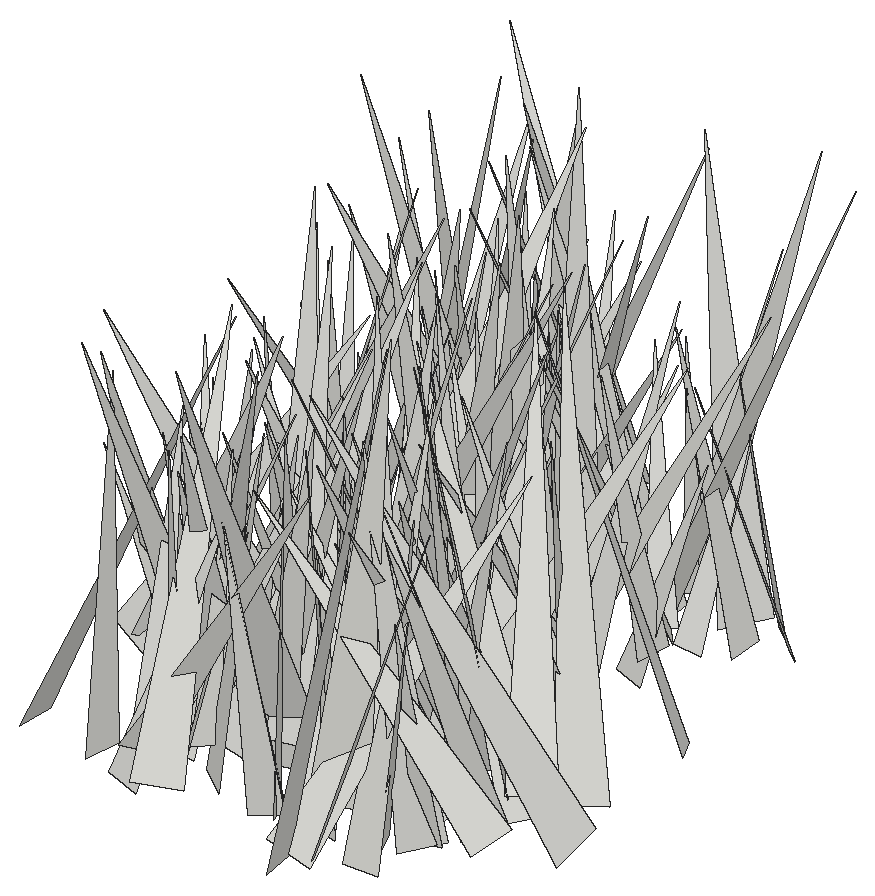
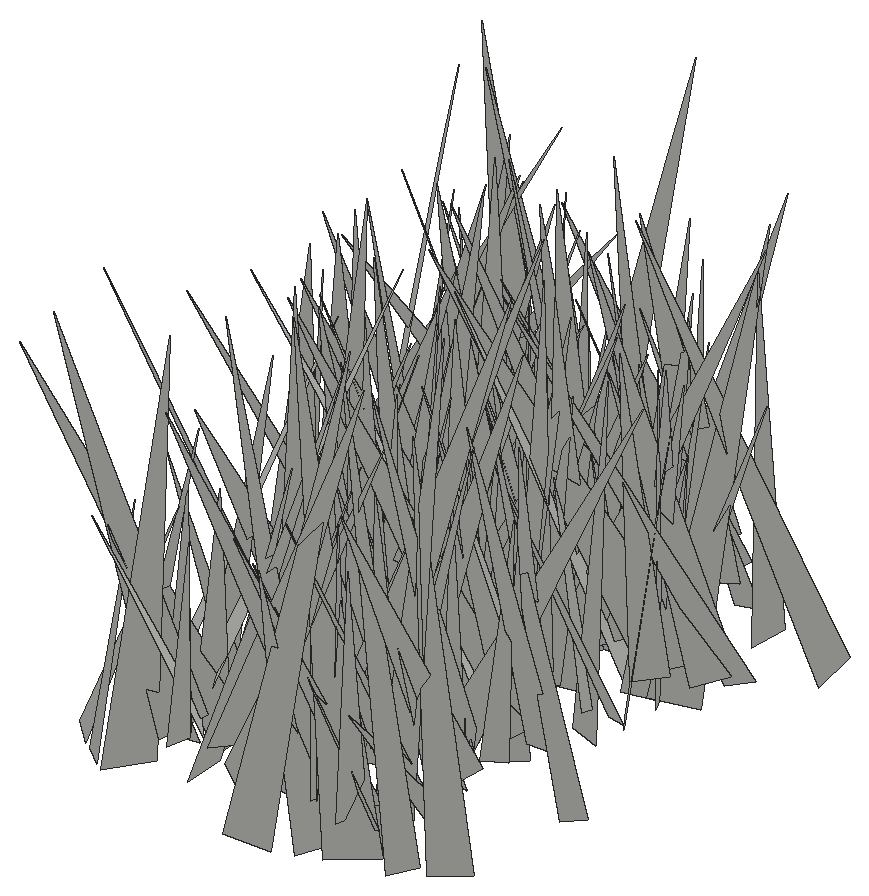
# SketchUp Ruby script. Lengths in inches.
U = 1.inch
M = Sketchup.active_model
def pt(a) = Geom::Point3d.new(a.map { |v| v * U })
def face(e, loops, mat)
  f = e.add_face(loops[0].map { |a| pt(a) })
  loops[1..].each { |l| e.add_face(l.map { |a| pt(a) }).erase! }
  f.material = f.back_material = mat if mat
  f
end
# faces: each face lists its corners as indices into pts; further lists are holes
def faces(e, pts, list, mat = nil) = list.each { |f| face(e, (f[0].is_a?(Array) ? f : [f]).map { |l| l.map { |i| pts[i] } }, mat) }
# xy, xz, yz: faces in a plane at the given z, y or x. An outline is a flat list of corners, or four numbers for a rectangle; further outlines are holes
def ring(l) = l.size == 4 ? [[l[0], l[1]], [l[2], l[1]], [l[2], l[3]], [l[0], l[3]]] : l.each_slice(2).to_a
def flat(e, list, mat, &to3) = list.each { |f| face(e, (f[0].is_a?(Array) ? f : [f]).map { |l| ring(l).map { |u, v| to3.(u, v) } }, mat) }
def xy(e, z, list, mat = nil) = flat(e, list, mat) { |x, y| [x, y, z] }
def xz(e, y, list, mat = nil) = flat(e, list, mat) { |x, z| [x, y, z] }
def yz(e, x, list, mat = nil) = flat(e, list, mat) { |y, z| [x, y, z] }
def lines(e, pts, list) = list.each { |a, b| e.add_line(pt(pts[a]), pt(pts[b])) }
# prism: a flat outline (further loops are holes) pulled along v
def prism(e, loops, v, mat = nil)
  f = face(e, loops, mat); d = Geom::Vector3d.new(v.map { |x| x * U })
  f.pushpull(f.normal.samedirection?(d) ? d.length : -d.length)
end
def box(e, o, s, mat = nil) = prism(e, [[o, [o[0] + s[0], o[1], o[2]], [o[0] + s[0], o[1] + s[1], o[2]], [o[0], o[1] + s[1], o[2]]]], [0, 0, s[2]], mat)
def at(x, y, z, deg = 0) = Geom::Transformation.translation(pt([x, y, z])) * Geom::Transformation.rotation(ORIGIN, Z_AXIS, deg.degrees)
def axes(o, x, y, z) = Geom::Transformation.new([*x, 0, *y, 0, *z, 0, *pt(o).to_a, 1])
def part(name) = M.definitions.add(name)
# library, detail: a bought-in or finely detailed component or shape, given as its bounding box
def library(name, o, s) = part(name).tap { |d| box(d.entities, o, s) }
def detail(e, o, s) = box(e.add_group.entities, o, s)
def put(e, d, t, mat = nil) = e.add_instance(d, t).tap { |i| i.material = mat if mat }
def group(e, t, mat = nil) = e.add_group.tap { |g| g.transformation = t; g.material = mat if mat }.entities
root = M.entities
c1 = part("fur_instance\#9")
p = [[0.8125,0,1.79],[0.67,-0.02,1.48],[0,-0.11,0],[0,0.11,0]]
faces(c1.entities,p,[[0,1,2,3]])
put(root,c1,axes([124.61,121.58,-28.22],[-3.04551,1.64304,1.0176],[0.80196,2.80235,-2.12461],[1.7584,1.56764,2.73144]))
put(root,c1,axes([126.19,110.12,-28.22],[-4.64353,0.24048,0.81476],[0.40253,4.60984,0.93348],[0.74809,-0.98772,4.55508]))
put(root,c1,axes([122.36,107.19,-28.22],[7.61599,0.93725,0.32253],[0.89381,-7.57423,0.90437],[-0.42844,0.85927,7.61996]))
put(root,c1,axes([124.81,111.45,-28.22],[2.89826,-6.60565,0.55734],[-6.55377,-2.94663,-0.84295],[-0.99662,0.16719,7.16407]))
put(root,c1,axes([122.79,118.57,-28.22],[-0.06945,-5.66946,1.63507],[-5.27402,0.7929,2.5253],[2.64594,1.43164,5.07647]))
put(root,c1,axes([125.08,106.82,-28.22],[5.69837,-0.41307,2.53776],[-0.52377,-6.22748,0.16244],[-2.51724,0.36068,5.71101]))
put(root,c1,axes([125.2,113.25,-28.22],[-3.34648,-2.86729,1.25208],[-2.75468,3.56945,0.81158],[1.4835,0.16004,4.33146]))
put(root,c1,axes([126.88,119.04,-27.1],[0.00181,-5.98408,0.19016],[-5.68264,-0.06159,-1.88392],[-1.88493,0.17992,5.67979]))
put(root,c1,axes([123.53,123.28,-28.22],[2.30675,-6.01681,0.97122],[-6.03702,-2.11321,1.24701],[0.83643,1.34116,6.32203]))
put(root,c1,axes([124.8,117.43,-27.1],[0.44242,5.64748,1.29703],[5.78226,-0.34572,-0.46699],[0.37666,-1.32609,5.6455]))
put(root,c1,axes([125.51,120.32,-27.1],[-5.11664,3.91829,0.85035],[3.38571,4.96082,-2.48663],[2.14782,1.51438,5.94556]))
put(root,c1,axes([125.24,111.59,-28.22],[-4.21315,-2.34987,2.26772],[-2.4638,4.71684,0.31027],[2.14339,0.80291,4.81418]))
put(root,c1,axes([125.67,120.82,-28.22],[4.21835,1.12148,1.8478],[0.48542,-4.44001,1.58659],[-2.10629,1.22277,4.06632]))
put(root,c1,axes([125.59,114.58,-28.22],[-1.84582,-5.09705,1.94608],[-5.40108,1.99766,0.10933],[0.77171,1.78987,5.41987]))
put(root,c1,axes([125.86,111.73,-28.22],[1.70929,-4.46495,1.67991],[-4.63149,-1.98085,-0.55231],[-1.1433,1.34907,4.74893]))
put(root,c1,axes([125.46,118.85,-27.1],[2.03457,-2.99845,1.01926],[-3.06758,-2.16697,-0.25148],[-0.78708,0.69471,3.61482]))
put(root,c1,axes([124.99,112.33,-27.1],[3.66382,-3.28739,1.57998],[-3.52995,-3.75957,0.36325],[-0.918,1.33625,4.90903]))
put(root,c1,axes([126.52,115.62,-28.22],[-0.46142,6.00885,1.03301],[6.04976,0.32253,0.82618],[-0.75742,-1.08443,5.96964]))
put(root,c1,axes([126.78,108.91,-28.22],[-3.90269,-1.36809,1.23152],[-1.73858,3.68797,-1.41263],[0.60468,1.77384,3.88679]))
put(root,c1,axes([126.83,109.45,-27.1],[-3.66348,3.88372,0.60062],[3.90017,3.69385,-0.09601],[0.48235,-0.37054,5.33808]))
put(root,c1,axes([126.3,116.91,-28.22],[-2.6188,2.85202,1.01974],[2.95253,2.70449,0.01846],[0.67563,-0.76402,3.87193]))
put(root,c1,axes([124.25,114.82,-27.1],[2.1149,3.97719,0.39309],[3.90996,-1.96694,-1.13523],[0.82754,-0.87089,4.35914]))
put(root,c1,axes([125.79,123.23,-28.22],[-1.04012,-7.65192,1.88155],[-7.84849,1.17518,0.4406],[0.70237,1.80029,7.70971]))
put(root,c1,axes([128.03,119.93,-27.1],[-6.43885,-0.2283,0.73687],[-0.34147,6.39798,-1.00159],[0.69173,1.03328,6.36457]))
put(root,c1,axes([123.48,125.51,-27.1],[7.4678,0.08394,0.57516],[0.2355,-7.21321,-2.00499],[-0.53141,-2.01703,7.1941]))
put(root,c1,axes([123.48,111.28,-27.1],[4.4628,-4.8312,0.78242],[-4.8199,-4.15484,1.83716],[0.84924,1.80724,6.31521]))
put(root,c1,axes([126.61,123.95,-27.1],[-4.17339,1.81444,1.20525],[1.74242,4.34394,-0.50613],[1.30721,0.0026,4.52253]))
put(root,c1,axes([122.82,110.91,-27.1],[1.506,6.6666,0.93752],[6.04421,-0.91584,-3.19677],[2.9648,-1.51928,6.04088]))
put(root,c1,axes([124.81,111.29,-27.1],[3.82808,-2.96393,0.87418],[-3.08142,-3.76593,0.72521],[-0.23226,1.11183,4.78677]))
put(root,c1,axes([126.13,119.27,-27.1],[6.62272,2.03005,2.53711],[1.31072,-6.93962,2.13125],[-2.97322,1.46257,6.59085]))
put(root,c1,axes([127.06,109.6,-27.1],[1.34944,-6.66989,1.0863],[-6.57389,-1.5523,-1.36482],[-1.56569,0.76902,6.66676]))
put(root,c1,axes([128.25,112.76,-28.22],[-6.66712,2.68909,2.42043],[3.53397,5.92752,3.14894],[0.77508,-3.89533,6.46266]))
put(root,c1,axes([126.89,109.55,-28.22],[4.42222,0.57042,2.59632],[0.96066,-5.04183,-0.52855],[-2.47858,-0.93641,4.42741]))
put(root,c1,axes([126.93,106.68,-27.1],[-2.07994,4.49979,1.08625],[4.57933,2.1742,-0.23818],[0.67657,-0.88257,4.95151]))
put(root,c1,axes([126.49,119.4,-27.1],[0.16475,-3.83195,1.51207],[-4.1166,-0.0965,0.20397],[0.15418,1.51796,3.83006]))
put(root,c1,axes([124.79,121.87,-28.22],[2.64419,5.03318,0.33977],[4.95036,-2.51506,-1.26831],[0.97076,-0.88412,5.54221]))
put(root,c1,axes([125.23,114.86,-27.1],[4.19489,0.81761,0.41517],[0.91291,-3.90671,-1.53042],[-0.08632,-1.58339,3.99042]))
put(root,c1,axes([129.45,120.01,-27.1],[-0.93338,-7.69941,2.7531],[-7.87622,0.10215,-2.38461],[-2.19672,2.90522,7.38009]))
put(root,c1,axes([125.91,117.17,-27.1],[4.66394,-1.20705,1.00362],[-1.36601,-4.67089,0.73033],[-0.77347,0.97077,4.76192]))
put(root,c1,axes([126.33,119.3,-27.1],[2.59266,-2.6088,0.97622],[-2.78019,-2.50569,0.68761],[-0.17141,1.18171,3.61316]))
put(root,c1,axes([126.4,123.89,-28.22],[2.97768,-2.23657,0.59018],[-2.29034,-2.98547,0.24174],[-0.32391,0.5494,3.71623]))
put(root,c1,axes([126.83,108.05,-28.22],[-0.69382,4.82103,0.91338],[4.82167,0.84094,-0.77604],[0.90996,-0.78004,4.80848]))
put(root,c1,axes([125.34,108.33,-28.22],[4.56915,3.9518,0.34933],[3.96081,-4.51383,-0.74378],[0.22516,-0.79028,5.99505]))
put(root,c1,axes([126.96,109.85,-27.1],[3.0521,-3.8403,0.46149],[-3.78154,-3.08617,-0.67208],[-0.8129,-0.06212,4.85917]))
put(root,c1,axes([128.1,120.41,-27.1],[-0.91047,5.0165,1.03079],[5.11456,0.83694,0.44447],[-0.2628,-1.09133,5.07905]))
put(root,c1,axes([127.37,114.76,-27.1],[5.69628,-2.00129,2.37758],[-1.98509,-6.1627,-0.4314],[-2.39112,0.34864,6.02217]))
put(root,c1,axes([127.39,123.42,-27.1],[4.14484,0.5886,1.74948],[0.68446,-4.48393,-0.11303],[-1.71425,-0.36717,4.1849]))
put(root,c1,axes([129.4,118.64,-28.22],[-1.28539,6.13898,3.44989],[6.89976,0.39684,1.86462],[-1.40785,-3.66012,5.98853]))
put(root,c1,axes([127.125,110.68,-28.22],[6.25178,5.32919,0.93445],[4.93149,-6.20008,2.36594],[-2.22574,1.23164,7.86685]))
put(root,c1,axes([128.85,110.96,-28.22],[-5.31707,5.30249,0.96243],[5.27581,5.39738,-0.58989],[1.09932,-0.2564,7.48596]))
put(root,c1,axes([128.19,115.38,-28.22],[1.47343,-6.07806,1.78682],[-6.21699,-1.74005,-0.79238],[-1.21846,1.52838,6.20371]))
put(root,c1,axes([128.37,113.5,-28.22],[0.55696,-4.64877,2.01019],[-4.98122,-0.86859,-0.62855],[-0.91614,1.89648,4.63963]))
put(root,c1,axes([126.89,121.04,-28.22],[4.28943,0.41298,0.87796],[0.18379,-4.25331,1.1028],[-0.95267,1.03894,4.16576]))
put(root,c1,axes([127.2,114.43,-27.1],[4.74802,-2.11154,0.82126],[-1.70244,-4.58339,-1.94189],[-1.49491,-1.48682,4.81989]))
put(root,c1,axes([127.65,107.01,-27.1],[-2.05605,-4.2865,1.82271],[-4.5186,2.31917,0.35698],[1.13077,1.47345,4.74068]))
put(root,c1,axes([128.4,107.31,-27.1],[-3.95695,1.67084,0.9926],[1.45221,4.03835,-1.00857],[1.29152,0.5783,4.17516]))
put(root,c1,axes([125.59,124.08,-27.1],[2.92691,3.10527,0.26779],[2.82947,-2.4932,-2.01476],[1.3071,-1.55642,3.76168]))
put(root,c1,axes([128.03,126.96,-27.1],[0.49777,-7.47829,0.86543],[-7.52286,-0.52678,-0.22508],[-0.28353,0.84808,7.49146]))
put(root,c1,axes([127.15,109.96,-27.1],[3.45501,-4.88886,0.26504],[-4.85303,-3.46254,-0.60598],[-0.64754,-0.13474,5.95575]))
put(root,c1,axes([127.22,111.4,-27.1],[3.70956,-2.15387,1.10856],[-2.28011,-3.78925,0.26761],[-0.81802,0.79458,4.28116]))
put(root,c1,axes([125.91,110.67,-27.1],[7.47799,-1.52657,1.95795],[-2.25093,-6.79047,3.30259],[-1.04752,3.69369,6.88067]))
put(root,c1,axes([126.67,105.75,-28.22],[0.90877,4.85728,1.17196],[4.86719,-0.59112,-1.32422],[1.13009,-1.36012,4.76083]))
put(root,c1,axes([126.31,124.25,-28.22],[3.42079,-7.2545,1.9343],[-7.49487,-3.17419,1.34998],[0.44283,2.31686,7.90614]))
put(root,c1,axes([128.91,114.62,-27.1],[3.32641,-4.64571,1.36805],[-4.19977,-3.59363,-1.99171],[-2.41165,-0.14974,5.35544]))
put(root,c1,axes([126.58,115.8,-27.1],[4.75078,2.28793,0.55209],[2.32197,-4.75936,-0.25743],[-0.38451,-0.47246,5.26671]))
put(root,c1,axes([129.28,121.19,-27.1],[-7.73279,0.49202,2.83462],[1.75633,7.24586,3.53356],[2.27869,-3.91518,6.89581]))
put(root,c1,axes([128.625,110.95,-27.1],[-5.59489,5.13542,2.2708],[5.22691,5.9344,-0.54239],[2.05147,-1.11455,7.57503]))
put(root,c1,axes([126.5,119.03,-28.22],[2.82445,3.52777,0.66946],[3.53756,-2.58781,-1.2883],[0.61561,-1.31488,4.33162]))
put(root,c1,axes([128.8,104.64,-27.1],[-3.78371,6.02543,0.57396],[5.96039,3.82698,-0.88298],[1.05307,-0.01122,7.05993]))
put(root,c1,axes([126.0625,110.67,-27.1],[7.05622,-1.23215,0.51957],[-1.10047,-6.93599,-1.50315],[-0.75967,-1.39725,7.0035]))
put(root,c1,axes([128.875,119.2,-28.22],[-1.66344,3.87519,0.54462],[3.91265,1.65754,0.1564],[0.06977,-0.56232,4.21422]))
put(root,c1,axes([126.64,123.1,-27.1],[0.2906,4.64928,0.9365],[4.41539,0.07727,-1.75374],[1.73123,-0.9775,4.31562]))
put(root,c1,axes([130.64,124.34,-27.1],[-3.35511,-5.27651,0.83113],[-5.27558,3.11951,-1.49198],[-0.83701,1.48869,6.07225]))
put(root,c1,axes([129.95,111.08,-27.1],[-0.88602,-4.48963,1.06047],[-4.46813,0.56653,-1.33464],[-1.14769,1.26043,4.37728]))
put(root,c1,axes([131.8125,122.66,-27.1],[-7.18183,4.15456,0.03319],[4.14203,7.15453,0.70461],[-0.3242,-0.62648,8.26695]))
put(root,c1,axes([127.08,108.27,-27.1],[2.4518,5.85296,0.01413],[5.81055,-2.43218,-0.76857],[0.70347,-0.30989,6.29903]))
put(root,c1,axes([128.24,123.75,-28.22],[2.79226,2.81825,2.22878],[3.51982,-2.71249,-0.9798],[-0.72174,-2.32521,3.84438]))
put(root,c1,axes([129.82,122.47,-28.22],[-0.8094,5.47668,0.09308],[5.43232,0.79056,0.72297],[-0.70181,-0.19701,5.48875]))
put(root,c1,axes([130.74,116.34,-27.1],[-5.03149,-1.83162,1.20846],[-2.18082,4.50919,-2.24552],[0.24343,2.5384,4.86091]))
put(root,c1,axes([130.96,121,-28.22],[-2.36065,-3.34559,0.0438],[-3.13879,2.19578,-1.44709],[-1.15883,0.86782,3.83035]))
put(root,c1,axes([131.56,110.85,-28.22],[-6.207,1.9177,0.03314],[1.91765,6.20287,0.22937],[-0.03607,-0.22893,6.49244]))
put(root,c1,axes([128.375,106.45,-27.1],[2.97809,2.23148,0.68885],[2.24903,-3.04112,0.12836],[-0.62921,-0.30835,3.71915]))
put(root,c1,axes([129.11,114.62,-27.1],[-3.597,-0.64897,1.74683],[-0.97146,3.89365,-0.55385],[1.59023,0.91068,3.61287]))
put(root,c1,axes([128.09,123.63,-27.1],[4.34491,0.59069,1.09524],[0.90101,-4.23706,-1.28924],[-0.85828,-1.45776,4.19106]))
put(root,c1,axes([127.49,116.13,-27.1],[-1.94232,7.80928,1.11049],[7.41359,2.19794,-2.48968],[2.69386,-0.41817,7.65238]))
put(root,c1,axes([128.64,107.39,-28.22],[3.29579,4.51514,1.8086],[4.80118,-3.36974,-0.33663],[-0.7786,-1.66678,5.57991]))
put(root,c1,axes([130.25,108.91,-27.1],[-1.2461,7.24945,1.28302],[7.36015,1.19663,0.38699],[-0.1701,-1.32928,7.34558]))
put(root,c1,axes([128.07,109.08,-28.22],[0.38295,8.08113,1.09098],[7.9956,-0.1576,-1.6392],[1.60161,-1.14545,7.92239]))
put(root,c1,axes([130.41,113.375,-28.22],[2.49829,3.83803,2.30798],[4.11646,-3.0089,0.54773],[-1.76409,-1.58579,4.54664]))
put(root,c1,axes([128.87,110.87,-27.1],[-0.89521,-5.51634,1.09126],[-5.41102,1.14576,1.35291],[1.53027,0.82431,5.42227]))
put(root,c1,axes([128.0625,122.47,-27.1],[6.72656,-0.08852,1.07497],[-0.40385,-6.50233,1.99163],[-1.00015,2.03024,6.42556]))
put(root,c1,axes([130.95,113.4,-27.1],[-4.49131,4.50007,0.95246],[4.50728,4.57122,-0.34355],[0.91773,-0.42777,6.34858]))
put(root,c1,axes([127.1,106,-27.1],[4.74645,-3.63152,0.20608],[-3.44873,-4.38539,2.15263],[1.15614,1.82746,5.57521]))
put(root,c1,axes([127.26,116.85,-27.1],[5.75926,3.61485,0.22209],[3.58079,-5.62103,-1.36658],[0.54262,-1.27375,6.66098]))
put(root,c1,axes([131.33,121.13,-27.1],[-3.91396,0.19988,0.40503],[0.19284,3.93443,-0.07818],[0.40843,0.05784,3.91828]))
put(root,c1,axes([131.76,116.04,-28.22],[-5.84783,-0.54956,0.92386],[-0.66437,5.86496,-0.71656],[0.84507,0.80798,5.82972]))
put(root,c1,axes([130.01,109.39,-27.1],[2.00321,-7.73932,0.37509],[-7.71802,-2.02729,-0.61059],[-0.68548,0.20889,7.97102]))
put(root,c1,axes([130.5,121.49,-27.1],[1.64686,-6.77743,3.62945],[-7.62252,-1.92308,-0.13234],[-1.0018,3.49096,6.97339]))
put(root,c1,axes([129.75,118.65,-28.22],[5.65388,1.0827,1.74004],[0.6959,-5.81697,1.3583],[-1.92762,1.07564,5.59407]))
put(root,c1,axes([131.56,119.54,-27.1],[-4.31752,-0.25034,0.73123],[-0.52227,4.00392,-1.71296],[0.56974,1.77322,3.97108]))
put(root,c1,axes([130.98,123.25,-27.1],[-4.32918,-1.79601,0.73607],[-1.48596,4.22424,1.56749],[1.24875,-1.19977,4.41706]))
put(root,c1,axes([127.28,114.96,-28.22],[7.23014,-2.66142,0.8801],[-2.79977,-6.73645,2.62947],[0.1379,2.76941,7.24182]))
put(root,c1,axes([128.71,118.24,-28.22],[2.07554,-6.96607,1.71735],[-7.11885,-1.77704,1.39545],[0.89291,2.02467,7.13349]))
put(root,c1,axes([131.2,121.2,-28.22],[-4.34694,-0.07841,1.0456],[-0.20123,4.43859,-0.5037],[1.02905,0.53671,4.31837]))
put(root,c1,axes([132.1875,112.76,-28.22],[-2.43952,-3.83837,0.4143],[-3.75379,2.24378,-1.31547],[-0.90209,1.04325,4.3536]))
put(root,c1,axes([132.65,115.6,-28.22],[-1.18961,5.30841,0.21099],[4.92708,1.02155,2.07828],[-1.98686,-0.64508,5.02744]))
put(root,c1,axes([127.51,124.56,-28.22],[7.87771,-0.03675,0.30438],[0.03502,-7.66773,-1.83222],[-0.30459,-1.83219,7.66177]))
put(root,c1,axes([129.25,109.21,-28.22],[3.13574,-5.33007,1.5739],[-5.55752,-3.01682,0.85589],[-0.02918,1.79133,6.12454]))
put(root,c1,axes([130.51,110.9,-27.1],[4.15283,1.56186,1.94961],[1.7605,-4.5132,-0.13443],[-1.7723,-0.82343,4.43479]))
put(root,c1,axes([132.83,122.92,-28.22],[-7.49054,-0.65717,0.9559],[-0.61994,7.54719,0.33069],[0.98046,-0.24861,7.51203]))
put(root,c1,axes([131.02,106.84,-28.22],[1.81609,-4.28388,1.69446],[-4.45246,-2.09973,-0.53642],[-1.18256,1.32684,4.62191]))
put(root,c1,axes([128.34,110.23,-28.22],[3.82304,5.79974,2.60132],[6.29108,-3.01834,-2.51622],[0.9089,-3.50316,6.47466]))
put(root,c1,axes([131.23,107.0625,-28.22],[-4.01098,-1.65554,1.8183],[-2.11594,4.09606,-0.93811],[1.25294,1.61753,4.23659]))
put(root,c1,axes([131.26,115.2,-27.1],[0.92373,-7.0899,2.33425],[-7.39568,-1.18748,-0.68009],[-1.00963,2.21177,7.11741]))
put(root,c1,axes([131.72,116.18,-28.22],[-5.54219,0.95074,1.40051],[0.80502,5.69802,-0.68242],[1.48905,0.4581,5.58158]))
put(root,c1,axes([129.34,119.56,-28.22],[3.37968,-7.43588,1.46776],[-7.57694,-3.27406,0.85991],[0.19143,1.6903,8.12251]))
put(root,c1,axes([131.99,113.73,-27.1],[-3.10911,-5.59083,0.18925],[-5.58666,3.11434,0.22319],[0.28707,0.05678,6.39328]))
put(root,c1,axes([131.01,116.17,-28.22],[-2.23012,3.65012,0.738],[3.54975,2.34365,-0.86487],[1.12574,-0.15918,4.18913]))
put(root,c1,axes([131.86,106.82,-28.22],[-3.55733,-3.55392,1.20149],[-3.66341,3.64755,-0.05732],[0.80828,0.89081,5.02808]))
put(root,c1,axes([131.3,109.84,-27.1],[-1.57636,3.66287,0.67143],[3.67727,1.64614,-0.34684],[0.58749,-0.47537,3.97256]))
put(root,c1,axes([132.71,109.07,-27.1],[-5.22043,-0.84385,1.05571],[-1.17009,4.93002,-1.84535],[0.67639,2.01552,4.95577]))
put(root,c1,axes([128.96,121.53,-27.1],[4.72114,-1.50275,0.05764],[-1.46013,-4.53503,1.361],[0.36002,1.31378,4.76394]))
put(root,c1,axes([130.72,116.06,-27.1],[-2.364,-4.99525,1.36106],[-4.8414,2.66304,1.36474],[1.83462,0.59091,5.35523]))
put(root,c1,axes([133.125,121.79,-28.22],[-5.82181,0.2065,0.70872],[0.14567,5.84473,-0.50632],[0.72368,0.48471,5.80343]))
put(root,c1,axes([132.61,107.1,-28.22],[-2.1836,4.82414,0.14178],[4.82373,2.17653,0.23433],[-0.15514,-0.2257,5.29014]))
put(root,c1,axes([131.54,117.29,-27.1],[2.89571,-2.97183,2.13904],[-3.49598,-3.05481,0.48854],[-1.08874,1.90494,4.12046]))
put(root,c1,axes([132.45,117.67,-27.1],[0.36283,-7.33481,3.26148],[-7.98321,-0.67122,-0.62142],[-0.83968,3.21222,7.31744]))
put(root,c1,axes([131.44,109.26,-28.22],[4.8829,2.83209,2.83107],[3.60518,-5.05239,-1.16384],[-1.7431,-2.51617,5.52349]))
put(root,c1,axes([130.13,110.27,-28.22],[4.16572,3.95636,0.93283],[4.06431,-4.03236,-1.04767],[0.06588,-1.40123,5.64875]))
put(root,c1,axes([132.47,115.79,-27.1],[-2.78795,6.31949,0.96814],[6.36227,2.84625,-0.25738],[0.62828,-0.78026,6.90234]))
put(root,c1,axes([133.91,112.78,-28.22],[-6.81045,0.95525,0.6863],[0.79996,6.71798,-1.4123],[0.86231,1.31226,6.73054]))
put(root,c1,axes([131.15,111.29,-28.22],[3.63637,-5.76719,3.12725],[-6.51934,-3.57646,0.98508],[-0.73369,3.19558,6.74635]))
put(root,c1,axes([131.625,113.86,-27.1],[0.51611,-4.80053,1.29544],[-4.96034,-0.40702,0.46794],[0.34389,1.33374,4.80546]))
put(root,c1,axes([132.9375,115.5625,-28.22],[-0.49716,-5.04462,0.80589],[-5.07325,0.39247,-0.67299],[-0.59982,0.86174,5.02418]))
put(root,c1,axes([134.57,120.77,-27.1],[-5.605,-5.08718,0.25266],[-5.09303,5.60246,-0.18084],[0.06544,0.30374,7.56721]))
put(root,c1,axes([130.66,114.01,-27.1],[5.97415,4.42308,0.10738],[4.35531,-5.91092,1.16532],[-0.77872,0.87356,7.3414]))
put(root,c1,axes([131.17,119.5,-28.22],[0.97735,4.73028,0.44464],[4.65378,-0.86171,-1.06216],[0.95682,-0.64061,4.71196]))
put(root,c1,axes([133.18,109.45,-27.1],[-6.12251,3.37612,2.03098],[3.42132,6.417,-0.35327],[1.95387,-0.65732,6.98272]))
put(root,c1,axes([135.19,110.2,-28.22],[-5.14523,1.96025,0.06602],[1.88898,4.90265,1.64806],[-0.52792,-1.56261,5.25356]))
put(root,c1,axes([133.22,123.62,-27.1],[3.01506,-0.72225,2.0256],[-1.00024,-3.559,0.21985],[-1.90373,0.72607,3.09256]))
put(root,c1,axes([131.99,107.87,-28.22],[5.47327,5.90798,0.9862],[5.7796,-5.55993,1.23167],[-1.57262,0.12835,7.95889]))
put(root,c1,axes([133.1,112.39,-27.1],[2.61621,-5.42084,0.25429],[-5.22177,-2.59146,-1.52055],[-1.47757,-0.43991,5.82391]))
put(root,c1,axes([133.11,106.99,-28.22],[1.02394,3.35387,1.44831],[3.57422,-1.23084,0.32333],[-0.75567,-1.27715,3.49176]))
put(root,c1,axes([133.375,107.23,-27.1],[-3.75742,-0.36081,1.22113],[-0.40687,3.94545,-0.08619],[1.20657,0.20686,3.77372]))
put(root,c1,axes([134.76,110.41,-27.1],[-1.27388,-3.61865,0.59779],[-3.46584,0.98064,-1.44951],[-1.19998,1.0092,3.55195]))
put(root,c1,axes([133.32,117.68,-27.1],[-4.76497,-3.93422,0.44703],[-3.2824,4.31602,2.99679],[2.21445,-2.06803,5.40391]))
put(root,c1,axes([133.42,122.28,-27.1],[3.56764,3.88458,0.34534],[3.52617,-3.41301,1.96335],[-1.66594,1.09483,4.89523]))
put(root,c1,axes([133.62,110.93,-28.22],[-3.54385,2.2292,0.7922],[1.93522,3.55225,-1.33876],[1.36083,0.75365,3.96686]))
put(root,c1,axes([134.27,120.73,-27.1],[-2.51117,3.39602,0.58609],[3.43959,2.51478,0.1658],[0.21361,-0.57041,4.22035]))
put(root,c1,axes([131.54,112,-28.22],[7.1879,-0.3196,1.18159],[-0.53762,-7.14753,1.33717],[-1.09967,1.40532,7.06966]))
put(root,c1,axes([134.73,123.97,-28.22],[-6.40886,3.74132,2.19702],[3.96061,6.64492,0.23769],[1.77143,-1.32114,7.41717]))
put(root,c1,axes([132.78,113.35,-27.1],[4.609,-3.3139,0.05026],[-3.15306,-4.41083,-1.68231],[-1.0211,-1.33793,5.42168]))
put(root,c1,axes([133.09,104.79,-28.22],[7.46967,2.68884,2.29218],[2.3982,-7.79505,1.32883],[-2.59473,0.53597,7.82688]))
put(root,c1,axes([135.64,114.875,-27.1],[-5.10669,0.68056,0.36828],[0.71376,5.09217,0.48729],[0.29888,-0.53268,5.12875]))
put(root,c1,axes([133.66,123.13,-27.1],[1.81522,-3.21568,0.8696],[-3.29805,-1.87418,-0.04607],[-0.46866,0.73395,3.69235]))
put(root,c1,axes([134.68,113.25,-28.22],[-0.03159,-6.8611,0.78211],[-6.88005,-0.03586,-0.59249],[-0.59273,0.78192,6.83555]))
put(root,c1,axes([136.98,111.25,-28.22],[-3.78872,6.01371,0.63065],[5.87535,3.48538,2.06137],[-1.42923,-1.61377,6.8022]))
put(root,c1,axes([132.7,110.43,-27.1],[-1.98967,-4.65459,1.69235],[-4.24096,2.54317,2.00863],[2.55803,0.59592,4.64644]))
put(root,c1,axes([133.57,106.91,-27.1],[-3.8242,6.03816,3.67075],[6.53219,4.61268,-0.78232],[2.69524,-2.61192,7.10435]))
put(root,c1,axes([135.11,106.01,-28.22],[1.19903,6.87384,0.5978],[6.78552,-1.2847,1.16229],[-1.25048,-0.38022,6.88014]))
put(root,c1,axes([135.26,114.89,-28.22],[-6.0414,2.82747,0.77084],[2.14541,5.47009,-3.25002],[1.99649,2.67784,5.82499]))
put(root,c1,axes([134.34,112.89,-28.22],[4.86562,-4.5964,0.06859],[-4.19123,-4.47675,-2.68294],[-1.88818,-1.90726,6.13213]))
put(root,c1,axes([134.4,121.75,-28.22],[-0.04754,4.40868,0.34675],[4.41199,0.07095,-0.29716],[0.30179,-0.34273,4.39891]))
put(root,c1,axes([138.27,107.99,-27.1],[-5.02457,3.67244,0.21301],[3.24783,4.25941,3.17608],[-1.72736,-2.67378,5.35216]))
put(root,c1,axes([135.01,119.42,-27.1],[4.20178,-1.75309,2.00996],[-1.5081,-4.65512,-0.90755],[-2.19975,-0.15714,4.46146]))
put(root,c1,axes([136.22,109.66,-28.22],[-6.69372,-1.63538,1.73187],[-1.91789,6.76382,-1.02573],[1.41263,1.43387,6.81383]))
put(root,c1,axes([135.68,122.75,-28.22],[-5.16901,0.01394,1.37798],[0.15537,5.32107,0.52899],[1.36927,-0.55116,5.14189]))
put(root,c1,axes([132.17,114.36,-28.22],[1.42855,6.69806,0.59183],[6.31436,-1.12829,-2.47201],[2.31152,-1.05735,6.38701]))
put(root,c1,axes([133.64,122.85,-27.1],[6.60662,-2.19065,2.41659],[-2.83754,-6.55209,1.81792],[-1.6085,2.56075,6.71874]))
put(root,c1,axes([133.44,106.11,-28.22],[5.13146,2.31605,0.71954],[2.33013,-5.17519,0.0403],[-0.67253,-0.25897,5.62978]))
put(root,c1,axes([132.92,105.47,-28.22],[-1.51427,6.54379,0.36236],[5.84338,1.51647,-2.96661],[2.96773,0.35306,6.02606]))
put(root,c1,axes([135.69,108.1,-28.22],[4.51203,-4.20905,2.90182],[-4.30887,-5.21386,-0.8628],[-2.75143,1.26279,6.10984]))
put(root,c1,axes([137.97,117.19,-28.22],[-5.87124,-3.56524,0.53214],[-3.58838,5.68376,-1.51131],[-0.34307,1.5651,6.70063]))
put(root,c1,axes([133.56,120.72,-28.22],[7.63616,1.08232,1.22596],[0.61242,-7.3209,2.64853],[-1.51635,2.49367,7.24345]))
put(root,c1,axes([134.1,119.42,-28.22],[0.51441,-3.71167,1.78135],[-3.92489,0.09986,1.3415],[1.24297,1.85145,3.49879]))
put(root,c1,axes([135.88,124.18,-28.22],[-2.56443,-3.19615,1.19823],[-3.34404,2.653,-0.08027],[0.6845,0.98675,4.09698]))
put(root,c1,axes([137.68,108.73,-27.1],[-0.80032,5.57612,2.90873],[5.9333,-0.30294,2.21326],[-2.08561,-3.00158,5.18026]))
put(root,c1,axes([136.97,123.29,-28.22],[-2.96371,-3.18096,0.56073],[-3.21747,2.84043,-0.89238],[-0.28422,1.01488,4.25508]))
put(root,c1,axes([132.3125,118.38,-28.22],[4.59981,5.90875,0.46757],[5.722,-4.27232,-2.30133],[1.54616,-1.76752,7.12569]))
put(root,c1,axes([134.74,107.51,-28.22],[4.02483,1.17033,1.17041],[1.40502,-4.04247,-0.78939],[-0.87491,-1.10794,4.11653]))
put(root,c1,axes([135.67,108.375,-28.22],[0.76269,-3.95415,0.89534],[-4.04548,-0.80213,-0.09639],[-0.26648,0.86018,4.02588]))
put(root,c1,axes([137.45,110.85,-27.1],[-4.42637,5.44798,0.10976],[5.44745,4.42761,-0.08267],[0.13338,-0.03304,7.019]))
put(root,c1,axes([135.47,114.93,-27.1],[-4.30625,-1.78107,2.16646],[-1.55574,4.81995,0.87021],[2.33354,-0.07334,4.57807]))
put(root,c1,axes([139.09,110.82,-28.22],[-8.16776,0.06376,0.0825],[0.08376,7.86119,2.21763],[0.06209,-2.2183,7.8612]))
put(root,c1,axes([135.25,109.77,-27.1],[2.3418,4.95634,1.60959],[5.19702,-2.35112,-0.32146],[-0.38351,-1.59595,5.4723]))
put(root,c1,axes([136.63,114.48,-28.22],[0.09538,-4.31944,0.7575],[-4.29634,-0.24392,-0.84995],[-0.8791,0.72346,4.23607]))
put(root,c1,axes([137.7,112.83,-28.22],[-2.86004,7.00076,0.77945],[7.00763,2.7424,1.08181],[-0.71502,-1.12544,7.48466]))
put(root,c1,axes([136.4,111,-27.1],[-5.36571,-5.00333,1.81378],[-4.95811,5.63559,0.87824],[1.93398,0.5664,7.28374]))
